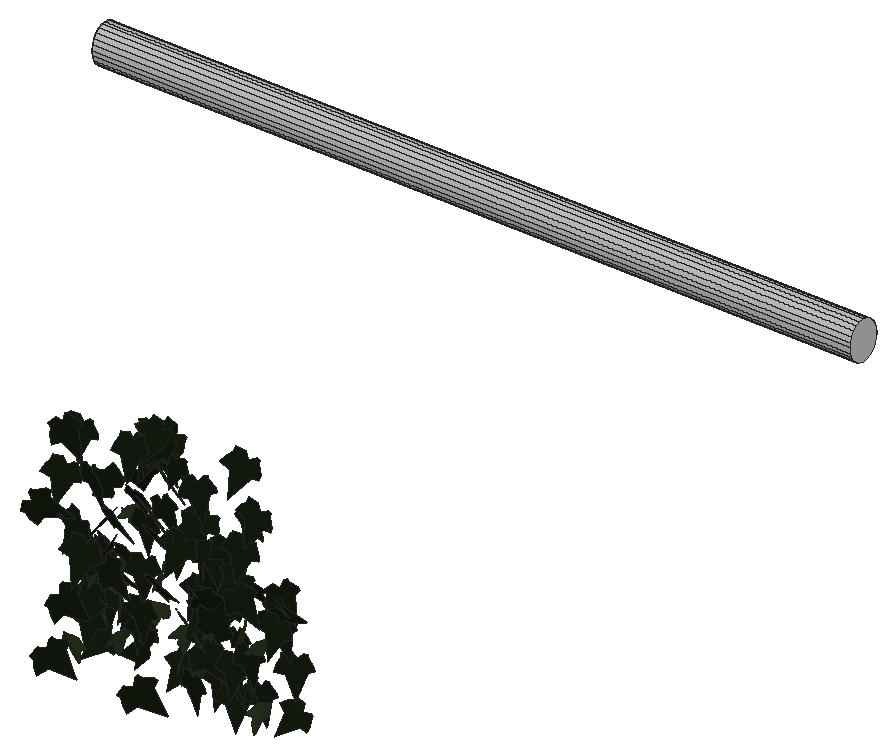
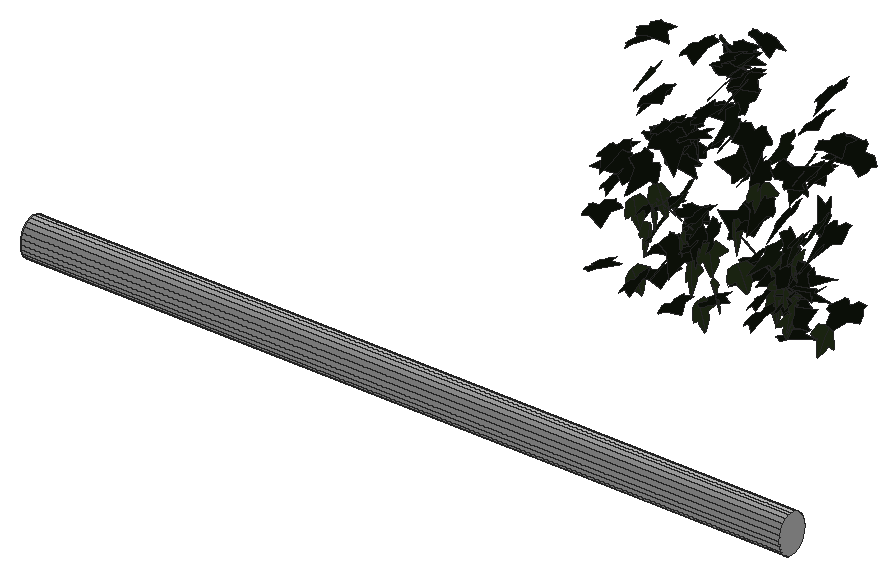
# SketchUp Ruby script. Lengths in inches.
U = 1.inch
M = Sketchup.active_model
def pt(a) = Geom::Point3d.new(a.map { |v| v * U })
def face(e, loops, mat)
  f = e.add_face(loops[0].map { |a| pt(a) })
  loops[1..].each { |l| e.add_face(l.map { |a| pt(a) }).erase! }
  f.material = f.back_material = mat if mat
  f
end
# faces: each face lists its corners as indices into pts; further lists are holes
def faces(e, pts, list, mat = nil) = list.each { |f| face(e, (f[0].is_a?(Array) ? f : [f]).map { |l| l.map { |i| pts[i] } }, mat) }
# xy, xz, yz: faces in a plane at the given z, y or x. An outline is a flat list of corners, or four numbers for a rectangle; further outlines are holes
def ring(l) = l.size == 4 ? [[l[0], l[1]], [l[2], l[1]], [l[2], l[3]], [l[0], l[3]]] : l.each_slice(2).to_a
def flat(e, list, mat, &to3) = list.each { |f| face(e, (f[0].is_a?(Array) ? f : [f]).map { |l| ring(l).map { |u, v| to3.(u, v) } }, mat) }
def xy(e, z, list, mat = nil) = flat(e, list, mat) { |x, y| [x, y, z] }
def xz(e, y, list, mat = nil) = flat(e, list, mat) { |x, z| [x, y, z] }
def yz(e, x, list, mat = nil) = flat(e, list, mat) { |y, z| [x, y, z] }
def lines(e, pts, list) = list.each { |a, b| e.add_line(pt(pts[a]), pt(pts[b])) }
# prism: a flat outline (further loops are holes) pulled along v
def prism(e, loops, v, mat = nil)
  f = face(e, loops, mat); d = Geom::Vector3d.new(v.map { |x| x * U })
  f.pushpull(f.normal.samedirection?(d) ? d.length : -d.length)
end
def box(e, o, s, mat = nil) = prism(e, [[o, [o[0] + s[0], o[1], o[2]], [o[0] + s[0], o[1] + s[1], o[2]], [o[0], o[1] + s[1], o[2]]]], [0, 0, s[2]], mat)
def at(x, y, z, deg = 0) = Geom::Transformation.translation(pt([x, y, z])) * Geom::Transformation.rotation(ORIGIN, Z_AXIS, deg.degrees)
def axes(o, x, y, z) = Geom::Transformation.new([*x, 0, *y, 0, *z, 0, *pt(o).to_a, 1])
def part(name) = M.definitions.add(name)
# library, detail: a bought-in or finely detailed component or shape, given as its bounding box
def library(name, o, s) = part(name).tap { |d| box(d.entities, o, s) }
def detail(e, o, s) = box(e.add_group.entities, o, s)
def put(e, d, t, mat = nil) = e.add_instance(d, t).tap { |i| i.material = mat if mat }
def group(e, t, mat = nil) = e.add_group.tap { |g| g.transformation = t; g.material = mat if mat }.entities
root = M.entities
M.materials.add("Glass Rail Metal").color = [192, 192, 192]
M.materials.add("efeu1").color = [18, 25, 13]
M.materials.add("efeu2").color = [43, 57, 29]
c1 = part("ivyleaf_10")
p = [[0,0.5,-0.03],[-0.0625,2.02,-0.43],[-0.19,2.01,-0.46],[-0.54,1.05,-0.29],[-0.52,0.625,-0.18],[-0.83,0.76,-0.28],
  [-1.16,0.64,-0.33],[-1.15,0.33,-0.24],[-0.77,-0.39,0.02],[-0.3,-0.51,0.16],[0.04,-0.48,0.23],[-0.02,2.01,-0.4375],
  [-0.06,2.01,-0.43],[0.04,-0.49,0.23],[0.67,-0.49,0.14],[1.38,0.36,-0.2],[1.375,0.51,-0.24],[0.81,0.65,-0.19],
  [0.62,0.59,-0.15],[0.6,1.09,-0.28],[0.5,1.23,-0.31]]
faces(c1.entities,p,[[0,1,2,3,4,5,6,7,8,9,10],[11,12,0,13,14,15,16,17,18,19,20]],"efeu2")
c2 = part("ivyleaf_9")
p = [[1.54,2.16,1.25],[1.36,2.04,1.19],[-0.21,0.99,0.68],[-0.71,1.11,0.82],[-0.85,0.86,0.67],[-0.8,0.17,0.21],
  [-0.9,-0.01,0.1],[-0.67,-0.16,-0.02],[-0.08,-0.08,-0.05],[-0.03,-0.6,-0.4],[0.65,-0.88,-0.66],[0.83,-0.6,-0.49],
  [1.29,-0.42,-0.43],[1.8125,-0.07,-0.26],[1.21,0.44,0.15]]
faces(c2.entities,p,[[0,1,2,3,4,5,6,7,8,9,10,11,12,13,14]],"efeu1")
prism(root,[[[506.55,180.51,322.8],[506.55,180.12,323.16],[506.55,179.8125,323.625],[506.55,179.625,324.17],[506.55,179.56,324.75],[506.55,179.625,325.34],[506.55,179.8125,325.88],[506.55,180.12,326.35],[506.55,180.51,326.71],[506.55,180.97,326.9375],[506.55,181.46,327.01],[506.55,181.95,326.9375],[506.55,182.41,326.71],[506.55,182.8,326.35],[506.55,183.1,325.88],[506.55,183.29,325.34],[506.55,183.36,324.75],[506.55,183.29,324.17],[506.55,183.1,323.625],[506.55,182.8,323.16],[506.55,182.41,322.8],[506.55,181.95,322.57],[506.55,181.46,322.49],[506.55,180.97,322.57]]],[89.11,0,0],"Glass Rail Metal")
put(root,c1,axes([550.75,121.33,303.9],[-1.20254,0.27266,-0.15968],[0.15464,-0.04009,-1.23305],[-0.27555,-1.21243,0.00486]))
put(root,c2,axes([550.29,123.83,313.14],[0.49111,-1.17298,-0.10556],[-0.0271,0.10309,-1.27155],[1.17741,0.49163,0.01477]))
put(root,c2,axes([551.73,124.83,306.68],[0.05623,0.11627,1.24014],[-1.08279,0.61816,-0.00886],[-0.61566,-1.07656,0.12885]))
put(root,c2,axes([550.65,122.97,315.28],[0.15124,-1.09967,0.65353],[0.2098,-0.62785,-1.10501],[1.26189,0.23618,0.10539]))
put(root,c2,axes([551.92,124.11,308.99],[-1.06809,-0.39065,0.51456],[-0.44861,-0.26698,-1.13387],[0.4649,-1.15512,0.08805]))
put(root,c1,axes([551.66,124.49,307.85],[-0.43704,0.90131,0.74431],[-0.34637,0.65909,-1.0015],[-1.11642,-0.55732,0.01934]))
put(root,c2,axes([550.51,116.04,320.74],[0.3474,0.07002,-1.38742],[0.82242,1.14223,0.26357],[1.11958,-0.86078,0.2369]))
put(root,c2,axes([551.46,119.58,323.14],[-0.66617,-1.12365,-0.14844],[0.05409,0.14047,-1.30605],[1.13212,-0.66789,-0.02495]))
put(root,c2,axes([551.35,122.28,326.43],[-0.15034,-1.30098,0.18184],[0.01456,-0.18467,-1.30916],[1.31354,-0.14686,0.03532]))
put(root,c2,axes([551.21,117.24,304.77],[0.08985,-0.64685,-1.26838],[0.01386,1.27124,-0.64732],[1.42373,0.02845,0.08634]))
put(root,c2,axes([551.99,124.43,307.41],[-0.45771,-1.03835,0.5097],[-0.18785,-0.47415,-1.13462],[1.14135,-0.49445,0.01766]))
put(root,c2,axes([552.6,124.08,311.26],[-0.04156,0.89421,-0.88564],[-0.34289,-0.86065,-0.85288],[-1.21095,0.21301,0.2719]))
put(root,c1,axes([551.9,124.72,306.67],[0.21274,1.2267,0.08282],[0.04003,0.0771,-1.24474],[-1.22884,0.21488,-0.02621]))
put(root,c1,axes([552.34,124.5625,309.1],[0.13347,-1.22043,0.23334],[0.12473,-0.22034,-1.22376],[1.23626,0.15399,0.09828]))
put(root,c2,axes([551.85,118.74,328.22],[0.44718,-1.16932,-0.66772],[-0.12852,0.66331,-1.24766],[1.34039,0.4537,0.10314]))
put(root,c1,axes([552.25,123.65,311.35],[0.25625,-0.69508,1.02635],[0.38497,-0.9516,-0.74058],[1.17827,0.46208,0.01876]))
put(root,c2,axes([552.01,123.98,313.65],[1.01264,-0.66498,-0.3712],[-0.23876,0.30923,-1.20532],[0.72318,1.03325,0.12183]))
put(root,c2,axes([551.9375,122.7,321.5],[0.57498,-1.16449,0.11352],[0.03712,-0.10826,-1.29863],[1.16943,0.57599,-0.01459]))
put(root,c2,axes([552.93,124.32,308.52],[-0.96942,-0.76437,0.22315],[-0.19751,-0.10977,-1.23401],[0.7714,-0.98869,-0.03552]))
put(root,c2,axes([553.29,121.9,308.75],[-0.74267,-0.36255,0.93567],[-0.81903,-0.45352,-0.82582],[0.57975,-1.10515,0.03194]))
put(root,c2,axes([553.65,123.56,320.0625],[-0.10155,-0.01248,1.28198],[-1.27889,0.09101,-0.10042],[-0.08974,-1.28277,-0.0196]))
put(root,c2,axes([551.99,119.92,314.47],[0.22929,-0.54167,1.24992],[0.44433,-1.16845,-0.58787],[1.28775,0.49961,-0.01972]))
put(root,c2,axes([553.1,123.91,304.08],[-0.953,-0.68747,0.39775],[-0.1772,-0.42158,-1.15321],[0.77423,-0.9427,0.22566]))
put(root,c2,axes([552.54,124.75,308.18],[0.07979,-1.23685,0.17262],[0.00556,-0.17262,-1.23941],[1.24882,0.07979,-0.00551]))
put(root,c1,axes([552.93,124.42,309.65],[-1.08804,-0.54443,-0.31019],[0.40736,-0.14231,-1.17909],[0.47611,-1.12241,0.29996]))
put(root,c2,axes([553.35,122.65,312.91],[0.05737,0.89717,0.94759],[0.11387,0.94144,-0.89824],[-1.29995,0.12206,-0.03686]))
put(root,c2,axes([552.84,121.67,307.11],[-0.30163,-1.17771,0.26312],[0.21122,-0.31856,-1.18369],[1.18812,-0.24235,0.27723]))
put(root,c2,axes([553.2,123.42,313.09],[-0.40981,-0.96574,0.72072],[-0.13865,-0.71841,-1.04148],[1.19702,-0.41384,0.12611]))
put(root,c1,axes([553.7,124.1,311.68],[-0.32215,-1.20135,0.21009],[0.01606,-0.22146,-1.24171],[1.21948,-0.31444,0.07186]))
put(root,c2,axes([552.91,124.09,311.05],[1.21627,-0.12651,0.31625],[0.31624,-0.01626,-1.22272],[0.12654,1.2566,0.01602]))
put(root,c2,axes([553.65,118.8,318.47],[-0.23709,-1.17557,0.72144],[-0.14351,-0.70702,-1.19924],[1.3718,-0.27714,-0.00077]))
put(root,c2,axes([553.53,116.23,311.73],[0.36519,-0.60364,-1.26842],[-0.31643,1.24155,-0.68196],[1.36863,0.44812,0.18078]))
put(root,c1,axes([554.32,123.88,307.68],[0.67057,-0.88088,-0.61803],[-0.13271,0.65496,-1.07749],[1.06785,0.63455,0.25419]))
put(root,c2,axes([553.71,124.64,312.91],[1.18147,-0.31642,-0.28454],[-0.13448,0.51904,-1.13554],[0.40373,1.09883,0.45445]))
put(root,c2,axes([555.3,119.74,318.06],[0.10564,1.06428,0.73257],[-0.1435,0.74013,-1.05458],[-1.28404,0.00484,0.17812]))
put(root,c2,axes([555.5625,124.17,317.47],[1.12307,0.36716,-0.46141],[-0.50523,0.08737,-1.16021],[-0.30405,1.21101,0.2236]))
put(root,c2,axes([555.27,125.21,306.16],[0.13916,-1.16899,-0.36772],[-0.01267,0.36869,-1.17687],[1.22539,0.13657,0.02959]))
put(root,c2,axes([555.9,117.03,317.38],[-0.6423,-1.26278,0.00781],[-0.00684,-0.00528,-1.41674],[1.26279,-0.64233,-0.0037]))
put(root,c1,axes([556.08,124.15,318.36],[-0.60285,-1.10895,-0.13622],[0.14429,0.07621,-1.25902],[1.10793,-0.61333,0.08985]))
put(root,c1,axes([556.1875,121.89,306.125],[-0.15366,-1.25855,-0.09653],[-0.00178,0.09746,-1.26782],[1.26224,-0.15307,-0.01354]))
put(root,c2,axes([555.78,124.26,307.4375],[0.20981,-1.21381,-0.13253],[-0.01474,0.13195,-1.23178],[1.22093,0.21018,0.0079]))
put(root,c2,axes([556.16,119.78,314.24],[0.73329,-0.95784,-0.80466],[-0.3638,0.72912,-1.19945],[1.1969,0.80844,0.12841]))
put(root,c2,axes([556.65,123.21,320.53],[1.11692,0.20437,-0.61418],[-0.60975,-0.07887,-1.13511],[-0.21723,1.2722,0.0283]))
put(root,c2,axes([557.7,122.98,323.34],[0.35711,1.22201,-0.28573],[-0.03725,-0.28662,-1.27238],[-1.25442,0.35639,-0.04356]))
put(root,c2,axes([556.95,118.88,320.5],[1.14445,-0.58439,-0.19228],[-0.10553,0.2136,-1.2773],[0.60609,1.14066,0.14067]))
put(root,c2,axes([558.1,122.9,313.92],[-0.2116,-1.2691,-0.15785],[0.0205,0.15661,-1.28661],[1.27872,-0.21252,-0.00549]))
put(root,c1,axes([558.78,123.89,308.86],[-0.78047,-0.88814,0.41455],[-0.10529,-0.45089,-1.16421],[0.97445,-0.76005,0.20624]))
put(root,c2,axes([558.45,122.59,318.78],[0.23158,-1.2597,0.25257],[0.0605,-0.24567,-1.28073],[1.28335,0.2389,0.01479]))
put(root,c1,axes([559.52,123.48,312.97],[0.3969,-1.14305,-0.37989],[-0.06373,0.37949,-1.20844],[1.20284,0.39728,0.06133]))
put(root,c2,axes([559.64,120.99,308.55],[-0.14826,-1.21767,0.33421],[0.07803,-0.3447,-1.22127],[1.26029,-0.12191,0.11493]))
put(root,c2,axes([559.89,122.1,328],[-0.42833,-1.24571,0.06565],[-0.01844,-0.06308,-1.31729],[1.24731,-0.42872,0.00307]))
put(root,c2,axes([560.22,121.84,327.43],[-0.6509,-1.13399,0.15797],[-0.09507,-0.12755,-1.30739],[1.14099,-0.65754,-0.01882]))
put(root,c2,axes([559.96,122.98,323.99],[1.19334,-0.48176,-0.21472],[-0.19911,0.08036,-1.28691],[0.48842,1.20983,-0.00002]))
put(root,c2,axes([559.85,121.86,329.3],[0.46172,-1.23913,0.05503],[0.26125,0.03976,-1.29685],[1.21253,0.46328,0.25847]))
put(root,c2,axes([560.08,122.72,326.56],[0.63885,-1.10904,-0.28179],[-0.061,0.28927,-1.27676],[1.14265,0.6355,0.08939]))
put(root,c2,axes([560.97,121.43,329.17],[-0.89834,-0.86425,0.44533],[-0.2156,-0.41415,-1.23866],[0.94804,-0.91314,0.1403]))
put(root,c2,axes([561.77,118.67,308.05],[-1.09188,0.8593,0.50876],[-0.42444,0.28303,-1.38895],[-0.90393,-1.17087,0.03764]))
put(root,c2,axes([559.91,122.18,312.34],[0.51456,-0.60474,0.99323],[0.80002,-0.60414,-0.78229],[0.84392,0.94143,0.136]))
put(root,c2,axes([560.5625,119.48,311.75],[0.06644,-1.30132,0.10693],[0.01268,-0.10642,-1.30299],[1.30564,0.06725,0.00721]))
put(root,c2,axes([560.98,117.59,329.98],[-0.96779,-0.59131,-0.696],[0.65226,0.26229,-1.1298],[0.63924,-1.16286,0.09908]))
put(root,c2,axes([561.71,122.43,328.47],[-1.20646,-0.52985,0.0606],[-0.03163,-0.07853,-1.31635],[0.53236,-1.20542,0.05912]))
put(root,c2,axes([560.3,121.3,318.23],[0.87,-0.61804,0.72556],[0.66584,-0.30878,-1.06143],[0.68196,1.08995,0.11072]))
put(root,c2,axes([560.92,122.02,321.6],[0.59802,-1.14853,-0.22201],[-0.02934,0.23454,-1.29235],[1.16942,0.59322,0.08111]))
put(root,c2,axes([561.85,120.66,329.96],[-1.09081,-0.73592,0.0469],[-0.03808,-0.02742,-1.31585],[0.73643,-1.09147,0.00143]))
put(root,c2,axes([562.07,122.23,329.04],[-0.83722,-0.91955,0.44513],[-0.28907,-0.33876,-1.24351],[0.97987,-0.88562,0.01348]))
put(root,c1,axes([562.15,123.37,305.56],[0.73573,-1.02372,0.03362],[0.02708,-0.02195,-1.26064],[1.02392,0.73617,0.00918]))
put(root,c2,axes([562.375,123.85,304.41],[-0.6669,-0.9572,0.41119],[-0.08698,-0.43536,-1.15454],[1.03814,-0.65137,0.16742]))
put(root,c2,axes([562.1,122.69,326.18],[-0.15992,-1.11113,0.65945],[0.12113,-0.67445,-1.10703],[1.2864,-0.07462,0.18622]))
put(root,c2,axes([563.42,120.24,329.64],[-1.17712,0.59332,-0.12824],[0.10119,-0.08409,-1.31787],[-0.59852,-1.1811,0.0294]))
put(root,c2,axes([562.08,116.4375,304.93],[0.08464,-0.49814,-1.31185],[0.48707,1.24295,-0.44055],[1.316,-0.42799,0.24743]))
put(root,c1,axes([563.3125,123.98,303.42],[-0.01787,-1.23895,0.12133],[0.00935,-0.12147,-1.23903],[1.24485,-0.01687,0.01104]))
put(root,c1,axes([563.39,122.5625,308.79],[-0.51481,-1.1581,0.09082],[0.00536,-0.10171,-1.26653],[1.16164,-0.51277,0.04609]))
put(root,c2,axes([562.26,118.22,322.88],[0.46704,-0.90512,1.01318],[0.70099,-0.75721,-0.99958],[1.16379,0.81933,0.19548]))
put(root,c1,axes([563.97,124.36,307.38],[0.1207,-1.20828,-0.25206],[0.06401,0.25905,-1.21113],[1.23263,0.10486,0.08758]))
put(root,c2,axes([563.93,124.0625,312.83],[-0.41373,-1.13917,0.34819],[-0.07903,-0.34154,-1.21129],[1.18857,-0.41924,0.04067]))
put(root,c2,axes([563.5,123.6,312.33],[0.8176,-0.99353,0.04486],[0.02844,-0.03469,-1.28669],[0.99413,0.8181,-0.00008]))
put(root,c2,axes([563.3,122.2,309.87],[0.83363,-0.81788,0.58413],[0.39437,-0.43186,-1.16749],[0.92445,0.92176,-0.02869]))
put(root,c2,axes([564.07,120.44,319.24],[0.00322,-1.27166,0.22516],[0.0435,-0.22492,-1.27096],[1.29071,0.01075,0.04227]))
put(root,c2,axes([564.84,122.8,310.74],[0.85312,0.19077,-0.95318],[-0.91602,-0.26668,-0.87323],[-0.32534,1.25109,-0.0408]))
put(root,c2,axes([564.87,123.63,320.76],[-0.76717,-0.96416,0.37609],[-0.00894,-0.46196,-1.20254],[1.03487,-0.71874,0.26842]))
put(root,c2,axes([564.72,123.37,309.02],[-0.07903,-1.21572,-0.26778],[0.03639,0.26594,-1.21815],[1.24433,-0.08499,0.01862]))
put(root,c2,axes([565.71,123.98,309.05],[0.28082,1.17689,0.39667],[0.00508,0.4056,-1.20696],[-1.24193,0.26777,0.08476]))
put(root,c2,axes([565.54,125.29,303.65],[-0.39,-1.1564,0.05245],[-0.02169,-0.04804,-1.22038],[1.15739,-0.39057,-0.0052]))
put(root,c1,axes([565.71,123.34,309.07],[0.3436,-1.10031,0.51908],[0.15563,-0.4952,-1.15271],[1.20661,0.3772,0.00086]))
put(root,c2,axes([566.11,120.64,321.07],[-0.63951,-0.52114,1.04747],[-0.57916,-0.8962,-0.79947],[1.01654,-0.83845,0.20349]))
put(root,c2,axes([566.14,122.64,312.16],[-1.07581,-0.66392,0.12963],[-0.10291,-0.08006,-1.2641],[0.66858,-1.08063,0.01401]))
put(root,c2,axes([566.27,118.34,320.9],[-0.87183,-0.98057,0.02283],[-0.00219,-0.0286,-1.31199],[0.98084,-0.87166,0.01736]))
put(root,c2,axes([567.14,124.58,313.13],[-1.07456,0.55809,0.33362],[-0.37389,-0.00314,-1.19901],[-0.53195,-1.12515,0.16883]))
put(root,c2,axes([565.9,122.91,314.04],[0.78325,-1.03521,-0.03],[-0.01698,0.02478,-1.29813],[1.03551,0.78344,0.00141]))
put(root,c2,axes([566.22,120.96,319.14],[-0.24779,-0.04645,-1.31287],[1.28426,-0.28978,-0.23213],[-0.27652,-1.30424,0.09833]))
put(root,c2,axes([566.69,120.76,308.58],[0.2773,-0.9616,-0.83083],[0.18711,0.87201,-0.9468],[1.25696,0.08234,0.32424]))
put(root,c1,axes([568.08,124.24,314.1],[-1.05243,0.07632,0.6807],[-0.68486,-0.13893,-1.04329],[0.0119,-1.24566,0.15806]))
put(root,c2,axes([567.66,123.74,312.71],[-0.63151,-0.9735,0.51755],[-0.05642,-0.56712,-1.13558],[1.10108,-0.5874,0.23865]))
put(root,c2,axes([568.0625,121.43,316.26],[-1.08688,-0.69454,-0.14713],[0.14012,0.05389,-1.28949],[0.69598,-1.09546,0.02985]))
put(root,c2,axes([567.6,118.8,327.36],[-0.09572,-1.27306,-0.38239],[0.0628,0.37862,-1.27623],[1.32776,-0.10969,0.03279]))
put(root,c2,axes([567.47,118.28,306.9375],[0.35312,-1.18551,0.29194],[0.04017,-0.29246,-1.2362],[1.22026,0.35269,-0.04378]))
put(root,c2,axes([568.39,121.91,318.9],[0.57985,0.98508,-0.65961],[-0.38907,-0.53548,-1.14173],[-1.11986,0.6961,0.05514]))
put(root,c2,axes([567.875,120.89,319.73],[-0.30638,-1.19122,-0.49837],[0.10729,0.48694,-1.22988],[1.2868,-0.32422,-0.01611]))
put(root,c2,axes([567.81,120.39,317.1875],[0.43147,-1.20473,-0.0909],[-0.02847,0.08636,-1.27966],[1.20782,0.4324,0.00231]))
put(root,c2,axes([568.21,123.04,306.01],[0.51692,-1.14167,-0.11825],[-0.01664,0.12223,-1.25275],[1.14766,0.51599,0.0351]))
put(root,c2,axes([568.49,121.97,320.13],[0.01805,-1.16167,-0.58868],[0.01036,0.58884,-1.16168],[1.30227,0.01142,0.0174]))
put(root,c2,axes([568.64,123.48,309.73],[0.65464,-1.07935,-0.0328],[-0.01512,0.0292,-1.26236],[1.07974,0.65481,0.00222]))
put(root,c2,axes([569.04,122.48,307.49],[-0.18613,-1.25282,0.03415],[-0.01088,-0.03291,-1.26655],[1.25324,-0.18635,-0.00593]))
put(root,c2,axes([569.42,122.52,304.54],[-0.42788,-1.25234,-0.27887],[0.12791,0.25086,-1.32284],[1.27662,-0.44487,0.03907]))
put(root,c2,axes([568.78,117.66,316.125],[0.35721,0.50424,-1.15056],[0.67243,0.93362,0.61793],[1.06108,-0.76141,-0.00426]))
put(root,c1,axes([570.08,122.41,311.32],[0.49137,-1.12747,-0.26784],[-0.01493,0.28474,-1.226],[1.15876,0.48177,0.09778]))
put(root,c2,axes([569.98,122.95,315.69],[1.25708,0.30324,-0.10345],[-0.11173,0.02233,-1.29226],[-0.30029,1.26113,0.04776]))
put(root,c2,axes([571.14,121.06,317.83],[-1.14292,-0.56393,0.28451],[-0.25808,-0.11993,-1.27446],[0.57651,-1.17168,-0.00648]))
put(root,c1,axes([570.91,122.28,308.18],[-1.03225,0.66362,0.3006],[-0.2821,0.11655,-1.22602],[-0.6717,-1.06879,0.05295]))
put(root,c2,axes([570.82,121.96,329.41],[-0.9305,-0.96735,-0.03453],[0.03686,0.01245,-1.34212],[0.96727,-0.93106,0.01792]))
put(root,c2,axes([570.37,124.66,304.2],[0.10801,-1.22719,-0.215],[-0.00975,0.21496,-1.23191],[1.24585,0.10807,0.00899]))
put(root,c2,axes([570.63,117.25,313.55],[-0.88489,0.35327,1.1592],[0.97944,-0.63675,0.94171],[0.71361,1.31199,0.14491]))
put(root,c2,axes([571.59,120.6875,321.5],[-0.36734,-1.27771,0.14771],[-0.02559,-0.14633,-1.32938],[1.28597,-0.3679,0.01574]))
put(root,c1,axes([571.91,122.88,303.33],[-0.18874,-1.12984,0.47136],[0.14016,-0.49374,-1.12735],[1.21617,-0.11844,0.20307]))
put(root,c2,axes([571.64,121.23,310.03],[0.17242,-1.25535,-0.14444],[-0.0257,0.14227,-1.26712],[1.26337,0.17422,-0.00606]))
put(root,c2,axes([571.61,121.71,323.41],[-0.09142,-1.04647,0.79155],[0.2135,-0.79476,-1.02606],[1.29463,0.05717,0.22511]))
put(root,c1,axes([572.32,122.35,310.46],[-0.27302,-1.21507,0.10633],[-0.04247,-0.09942,-1.24521],[1.21897,-0.27561,-0.01957]))
put(root,c2,axes([573.12,122.22,314.375],[0.41724,0.11418,-1.19805],[0.63166,1.05853,0.32087],[1.02438,-0.69922,0.29012]))
put(root,c2,axes([573.75,123.29,316.38],[0.11686,-1.03055,-0.76501],[-0.04005,0.76487,-1.03649],[1.28284,0.11775,0.03733]))
put(root,c2,axes([574.11,119.65,326.16],[-0.44224,-1.19771,0.44407],[-0.00858,-0.46713,-1.26846],[1.27735,-0.41781,0.14522]))
put(root,c2,axes([574.0625,122.82,313.04],[0.23303,-1.20813,-0.37403],[-0.03699,0.37366,-1.22996],[1.26417,0.23363,0.03296]))
put(root,c2,axes([574.14,116.47,319.05],[0.38557,-1.04531,-0.7256],[0.05589,0.77136,-1.08154],[1.27124,0.28313,0.26763]))
put(root,c2,axes([575.56,124.15,303.66],[-0.83513,-0.75422,0.51805],[-0.17189,-0.55958,-1.09178],[0.89871,-0.80789,0.27258]))
put(root,c2,axes([575.375,120.96,314.29],[-0.3325,-1.20454,0.19011],[-0.04693,-0.18427,-1.24958],[1.21855,-0.33577,0.00375]))
put(root,c2,axes([575.6,123.3,309.51],[-0.44719,-1.11859,-0.4356],[0.11392,0.4232,-1.2037],[1.19499,-0.45894,-0.04826]))
